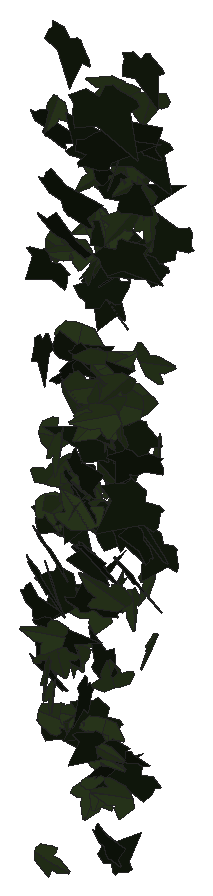
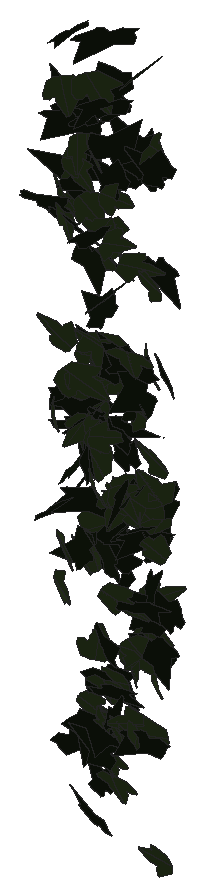
# SketchUp Ruby script. Lengths in inches.
U = 1.inch
M = Sketchup.active_model
def pt(a) = Geom::Point3d.new(a.map { |v| v * U })
def face(e, loops, mat)
  f = e.add_face(loops[0].map { |a| pt(a) })
  loops[1..].each { |l| e.add_face(l.map { |a| pt(a) }).erase! }
  f.material = f.back_material = mat if mat
  f
end
# faces: each face lists its corners as indices into pts; further lists are holes
def faces(e, pts, list, mat = nil) = list.each { |f| face(e, (f[0].is_a?(Array) ? f : [f]).map { |l| l.map { |i| pts[i] } }, mat) }
# xy, xz, yz: faces in a plane at the given z, y or x. An outline is a flat list of corners, or four numbers for a rectangle; further outlines are holes
def ring(l) = l.size == 4 ? [[l[0], l[1]], [l[2], l[1]], [l[2], l[3]], [l[0], l[3]]] : l.each_slice(2).to_a
def flat(e, list, mat, &to3) = list.each { |f| face(e, (f[0].is_a?(Array) ? f : [f]).map { |l| ring(l).map { |u, v| to3.(u, v) } }, mat) }
def xy(e, z, list, mat = nil) = flat(e, list, mat) { |x, y| [x, y, z] }
def xz(e, y, list, mat = nil) = flat(e, list, mat) { |x, z| [x, y, z] }
def yz(e, x, list, mat = nil) = flat(e, list, mat) { |y, z| [x, y, z] }
def lines(e, pts, list) = list.each { |a, b| e.add_line(pt(pts[a]), pt(pts[b])) }
# prism: a flat outline (further loops are holes) pulled along v
def prism(e, loops, v, mat = nil)
  f = face(e, loops, mat); d = Geom::Vector3d.new(v.map { |x| x * U })
  f.pushpull(f.normal.samedirection?(d) ? d.length : -d.length)
end
def box(e, o, s, mat = nil) = prism(e, [[o, [o[0] + s[0], o[1], o[2]], [o[0] + s[0], o[1] + s[1], o[2]], [o[0], o[1] + s[1], o[2]]]], [0, 0, s[2]], mat)
def at(x, y, z, deg = 0) = Geom::Transformation.translation(pt([x, y, z])) * Geom::Transformation.rotation(ORIGIN, Z_AXIS, deg.degrees)
def axes(o, x, y, z) = Geom::Transformation.new([*x, 0, *y, 0, *z, 0, *pt(o).to_a, 1])
def part(name) = M.definitions.add(name)
# library, detail: a bought-in or finely detailed component or shape, given as its bounding box
def library(name, o, s) = part(name).tap { |d| box(d.entities, o, s) }
def detail(e, o, s) = box(e.add_group.entities, o, s)
def put(e, d, t, mat = nil) = e.add_instance(d, t).tap { |i| i.material = mat if mat }
def group(e, t, mat = nil) = e.add_group.tap { |g| g.transformation = t; g.material = mat if mat }.entities
root = M.entities
M.materials.add("1026 AP 7946 SUNNY SIDE UP").color = [254, 231, 186]
M.materials.add("efeu1").color = [18, 25, 13]
M.materials.add("efeu2").color = [43, 57, 29]
c1 = part("ivyleaf_9")
p = [[1.54,2.16,1.25],[1.36,2.04,1.19],[-0.21,0.99,0.68],[-0.71,1.11,0.82],[-0.85,0.86,0.67],[-0.8,0.17,0.21],
  [-0.9,-0.01,0.1],[-0.67,-0.16,-0.02],[-0.08,-0.08,-0.05],[-0.03,-0.6,-0.4],[0.65,-0.88,-0.66],[0.83,-0.6,-0.49],
  [1.29,-0.42,-0.43],[1.8125,-0.07,-0.26],[1.21,0.44,0.15]]
faces(c1.entities,p,[[0,1,2,3,4,5,6,7,8,9,10,11,12,13,14]],"efeu1")
c2 = part("ivyleaf_10")
p = [[0,0.5,-0.03],[-0.0625,2.02,-0.43],[-0.19,2.01,-0.46],[-0.54,1.05,-0.29],[-0.52,0.625,-0.18],[-0.83,0.76,-0.28],
  [-1.16,0.64,-0.33],[-1.15,0.33,-0.24],[-0.77,-0.39,0.02],[-0.3,-0.51,0.16],[0.04,-0.48,0.23],[-0.02,2.01,-0.4375],
  [-0.06,2.01,-0.43],[0.04,-0.49,0.23],[0.67,-0.49,0.14],[1.38,0.36,-0.2],[1.375,0.51,-0.24],[0.81,0.65,-0.19],
  [0.62,0.59,-0.15],[0.6,1.09,-0.28],[0.5,1.23,-0.31]]
faces(c2.entities,p,[[0,1,2,3,4,5,6,7,8,9,10],[11,12,0,13,14,15,16,17,18,19,20]],"efeu2")
put(root,c1,axes([115.49,209.5,255.13],[-0.02705,-0.01002,-0.28667],[0.31242,-0.19569,-0.00654],[-0.30662,-0.19851,0.01862]),"1026 AP 7946 SUNNY SIDE UP")
put(root,c2,axes([114.77,209.6,259.99],[0.2251,-0.13197,0.25987],[0.25129,-0.19741,-0.2004],[0.37171,0.21338,-0.02189]),"1026 AP 7946 SUNNY SIDE UP")
put(root,c1,axes([114.3,209.47,257.21],[0.37652,-0.17867,-0.10207],[-0.14408,0.04077,-0.30679],[0.28627,0.25552,-0.02016]),"1026 AP 7946 SUNNY SIDE UP")
put(root,c1,axes([114.8,209.73,264.13],[0.4236,-0.17591,0.05148],[-0.04391,0.05014,0.33064],[-0.28462,-0.26955,0.02561]),"1026 AP 7946 SUNNY SIDE UP")
put(root,c1,axes([114.54,210.03,264.7],[-0.02289,-0.05893,0.36895],[0.34373,-0.28796,-0.0413],[0.45623,0.21399,0.04963]),"1026 AP 7946 SUNNY SIDE UP")
put(root,c1,axes([115.48,209.95,267.17],[-0.01242,-0.29597,-0.23302],[0.07302,0.22201,-0.3019],[0.57954,-0.03432,0.03305]),"1026 AP 7946 SUNNY SIDE UP")
put(root,c2,axes([114.04,210.18,254.74],[0.1255,-0.13859,0.23139],[0.21382,-0.18047,-0.16498],[0.3569,0.15685,0.01747]),"1026 AP 7946 SUNNY SIDE UP")
put(root,c2,axes([114.22,210.23,255.45],[-0.06096,-0.0694,-0.27227],[-0.3065,-0.17948,0.07708],[-0.30025,0.19731,-0.0234]),"1026 AP 7946 SUNNY SIDE UP")
put(root,c1,axes([115.21,209.97,265.93],[0.19681,0.10758,0.34086],[0.45934,0.1573,-0.16593],[-0.29545,0.31622,-0.03091]),"1026 AP 7946 SUNNY SIDE UP")
put(root,c2,axes([115.77,210.21,252.66],[0.15347,-0.06856,-0.24948],[-0.35736,0.08662,-0.11932],[0.16865,0.24593,-0.0258]),"1026 AP 7946 SUNNY SIDE UP")
put(root,c2,axes([115.29,210.39,260.32],[0.11174,0.03667,-0.27202],[-0.32658,-0.16404,-0.08195],[-0.2633,0.21903,-0.01379]),"1026 AP 7946 SUNNY SIDE UP")
put(root,c1,axes([116.04,210.45,258.76],[-0.41291,-0.14993,0.08346],[-0.08748,-0.06688,-0.31043],[0.25396,-0.26681,0.02877]),"1026 AP 7946 SUNNY SIDE UP")
put(root,c2,axes([115.51,210.35,256.59],[-0.27398,-0.02999,-0.24976],[-0.38052,-0.01791,0.18148],[-0.05045,0.29788,-0.01246]),"1026 AP 7946 SUNNY SIDE UP")
put(root,c1,axes([115.21,210.37,253.53],[0.09807,0.09154,-0.24899],[-0.17159,-0.21664,-0.11456],[-0.36922,0.12499,-0.01289]),"1026 AP 7946 SUNNY SIDE UP")
put(root,c2,axes([115.05,210.42,260.17],[0.26287,0.12848,-0.18106],[-0.19124,-0.12978,-0.21677],[-0.28504,0.20555,-0.02154]),"1026 AP 7946 SUNNY SIDE UP")
put(root,c2,axes([114.9,210.35,253.42],[-0.09458,-0.00259,-0.25397],[0.37678,-0.06028,-0.05993],[-0.09114,-0.24649,0.0158]),"1026 AP 7946 SUNNY SIDE UP")
put(root,c2,axes([114.94,210.43,263.36],[0.03486,-0.2653,-0.03718],[-0.00865,0.03424,-0.27405],[0.4206,0.02269,-0.00256]),"1026 AP 7946 SUNNY SIDE UP")
put(root,c1,axes([114.86,210.52,256.11],[0.33863,0.01352,0.15626],[-0.23931,0.02275,0.22076],[-0.00331,-0.26238,0.02564]),"1026 AP 7946 SUNNY SIDE UP")
put(root,c1,axes([115.53,210.38,263.84],[0.01179,-0.09483,-0.26226],[0.13606,0.24168,-0.0889],[0.40408,-0.07861,0.03759]),"1026 AP 7946 SUNNY SIDE UP")
put(root,c1,axes([115.07,210.59,251.21],[-0.02053,-0.0128,0.25407],[0.16189,-0.22485,-0.00772],[0.35309,0.10235,0.01831]),"1026 AP 7946 SUNNY SIDE UP")
put(root,c1,axes([113.72,210.6,254.33],[0.32164,-0.14094,-0.00848],[0.03041,0.01504,0.25487],[-0.21983,-0.20414,0.02286]),"1026 AP 7946 SUNNY SIDE UP")
put(root,c1,axes([113.82,210.49,255.3],[0.34152,0.05738,-0.19253],[0.26733,0.08346,0.23003],[0.15276,-0.27433,0.02789]),"1026 AP 7946 SUNNY SIDE UP")
put(root,c1,axes([113.64,210.67,256.93],[0.12988,-0.19391,0.19882],[0.1029,-0.18292,-0.21803],[0.41895,0.10504,-0.00808]),"1026 AP 7946 SUNNY SIDE UP")
put(root,c1,axes([115.83,210.7,257.8],[0.15212,-0.21561,-0.10881],[0.09876,-0.08582,0.24206],[-0.3635,-0.11354,0.02023]),"1026 AP 7946 SUNNY SIDE UP")
put(root,c1,axes([114.71,210.74,256.87],[0.1616,-0.23896,-0.11608],[0.08148,-0.09884,0.26727],[-0.40642,-0.11483,0.00743]),"1026 AP 7946 SUNNY SIDE UP")
put(root,c1,axes([113.84,210.53,262.95],[0.16397,0.01617,-0.24849],[-0.35536,-0.08702,-0.10713],[-0.13536,0.24804,-0.01975]),"1026 AP 7946 SUNNY SIDE UP")
put(root,c2,axes([113.72,210.74,254.05],[0.15207,-0.08677,0.24998],[0.24185,-0.18917,-0.13368],[0.32604,0.1808,-0.01744]),"1026 AP 7946 SUNNY SIDE UP")
put(root,c2,axes([114.01,210.55,254.86],[-0.26503,-0.20195,-0.05406],[0.07527,0.02672,-0.2701],[0.31887,-0.17415,0.01882]),"1026 AP 7946 SUNNY SIDE UP")
put(root,c1,axes([114.375,210.72,258.6],[-0.02097,0.02299,0.28356],[0.17416,-0.25185,0.02574],[0.39764,0.11152,0.00368]),"1026 AP 7946 SUNNY SIDE UP")
put(root,c2,axes([114.52,210.61,257.78],[0.28251,0.18577,0.10315],[-0.13701,-0.05295,0.26477],[0.30137,-0.19822,0.02368]),"1026 AP 7946 SUNNY SIDE UP")
put(root,c1,axes([113.3,210.73,255.48],[0.00996,0.00191,0.28312],[0.19716,-0.24462,-0.00265],[0.38452,0.12538,-0.00597]),"1026 AP 7946 SUNNY SIDE UP")
put(root,c1,axes([115.78,210.625,259.53],[0.14363,0.16281,-0.19678],[-0.11706,-0.17757,-0.19271],[-0.37804,0.11684,-0.01509]),"1026 AP 7946 SUNNY SIDE UP")
put(root,c1,axes([115.4,210.63,257.99],[0.19317,-0.16992,-0.17017],[-0.16403,0.12708,-0.21511],[0.3334,0.16097,-0.00723]),"1026 AP 7946 SUNNY SIDE UP")
put(root,c1,axes([113.93,210.66,255.84],[0.0528,-0.16787,0.18558],[-0.00367,0.18254,0.17583],[-0.38826,-0.02455,0.02358]),"1026 AP 7946 SUNNY SIDE UP")
put(root,c2,axes([114.875,210.75,253.59],[0.38898,0.00524,0.00305],[0.00537,-0.02319,-0.25391],[-0.00777,0.24631,-0.02251]),"1026 AP 7946 SUNNY SIDE UP")
put(root,c2,axes([114.84,210.8,260.14],[-0.24969,-0.2504,-0.08179],[-0.08858,-0.05646,0.30464],[-0.40276,0.16766,-0.0163]),"1026 AP 7946 SUNNY SIDE UP")
put(root,c1,axes([114.47,210.69,257.07],[0.39184,-0.07303,0.03452],[0.04122,-0.03074,-0.26675],[0.11973,0.24961,-0.02115]),"1026 AP 7946 SUNNY SIDE UP")
put(root,c1,axes([115.1,210.56,262.66],[-0.43965,0.1105,-0.05061],[-0.06013,0.03827,0.30917],[0.18082,0.28141,-0.02024]),"1026 AP 7946 SUNNY SIDE UP")
put(root,c2,axes([114.42,210.61,260.46],[-0.13007,-0.07676,0.26913],[0.25557,0.2057,0.1163],[-0.34432,0.18168,-0.01534]),"1026 AP 7946 SUNNY SIDE UP")
put(root,c2,axes([115.24,210.77,259.72],[-0.36298,0.15078,0.05464],[0.08607,-0.01136,0.28323],[0.23565,0.2364,-0.01929]),"1026 AP 7946 SUNNY SIDE UP")
put(root,c1,axes([113.37,210.9,260.95],[-0.14874,-0.02745,-0.25593],[0.37908,-0.0795,-0.08604],[-0.10277,-0.25351,0.05305]),"1026 AP 7946 SUNNY SIDE UP")
put(root,c2,axes([115.23,210.9,260.8],[-0.12716,-0.18939,0.17059],[-0.08336,-0.15835,-0.21281],[0.38783,-0.09613,0.01019]),"1026 AP 7946 SUNNY SIDE UP")
put(root,c2,axes([114.66,211,263.1],[0.01443,-0.03583,0.29115],[0.14207,-0.26801,-0.03957],[0.42515,0.09078,0.00334]),"1026 AP 7946 SUNNY SIDE UP")
put(root,c2,axes([113.38,210.89,250.3],[-0.0357,-0.01163,-0.24681],[0.32083,-0.12732,-0.0143],[-0.19808,-0.20413,0.02132]),"1026 AP 7946 SUNNY SIDE UP")
put(root,c1,axes([114.7,210.9,259.35],[-0.18541,-0.10774,-0.21597],[-0.24572,-0.13885,0.16372],[-0.27632,0.19576,-0.00067]),"1026 AP 7946 SUNNY SIDE UP")
put(root,c1,axes([115.65,210.9,267.59],[0.04255,-0.2644,-0.06219],[-0.01157,0.05842,-0.27346],[0.42576,0.02801,-0.00122]),"1026 AP 7946 SUNNY SIDE UP")
put(root,c1,axes([114.75,210.98,253.62],[-0.37392,-0.08956,0.05895],[-0.0713,-0.04271,-0.26091],[0.15162,-0.24095,0.02269]),"1026 AP 7946 SUNNY SIDE UP")
put(root,c2,axes([115.34,210.97,256.32],[0.2612,-0.09908,0.20455],[0.24482,-0.12567,-0.19896],[0.24974,0.22682,-0.0189]),"1026 AP 7946 SUNNY SIDE UP")
put(root,c1,axes([113.73,210.8125,254.89],[0.23732,0.07635,-0.22376],[-0.28899,-0.11732,-0.17439],[-0.21909,0.23744,-0.01234]),"1026 AP 7946 SUNNY SIDE UP")
put(root,c2,axes([114.68,211.01,259.58],[-0.02566,0.00037,0.29554],[0.36428,-0.16945,0.01281],[0.26604,0.23206,0.01097]),"1026 AP 7946 SUNNY SIDE UP")
put(root,c2,axes([114.05,210.97,254.79],[-0.22284,-0.18903,0.15562],[-0.10489,-0.13903,-0.24281],[0.36683,-0.15459,0.0251]),"1026 AP 7946 SUNNY SIDE UP")
put(root,c1,axes([113.85,211.07,267.32],[-0.01384,-0.29289,0.11753],[-0.00898,-0.11563,-0.30254],[0.49512,-0.01029,-0.0022]),"1026 AP 7946 SUNNY SIDE UP")
put(root,c2,axes([114.27,210.8,257.76],[0.03886,-0.25967,0.13505],[-0.02362,0.13174,0.26948],[-0.45784,-0.02884,-0.00244]),"1026 AP 7946 SUNNY SIDE UP")
put(root,c1,axes([113.9375,211.03,260.02],[0.11703,-0.16173,0.19744],[0.10624,-0.18058,-0.1842],[0.38088,0.10006,-0.00928]),"1026 AP 7946 SUNNY SIDE UP")
put(root,c1,axes([115.42,210.98,265.85],[-0.14077,0.00313,0.31162],[0.29124,-0.24882,0.05768],[0.37604,0.19388,0.07199]),"1026 AP 7946 SUNNY SIDE UP")
put(root,c1,axes([115.99,210.93,263.52],[-0.41705,0.07773,0.04163],[-0.07052,-0.01141,-0.28378],[-0.11797,-0.26798,0.02245]),"1026 AP 7946 SUNNY SIDE UP")
put(root,c1,axes([115.45,210.78,258.78],[0.06346,-0.01232,-0.27237],[-0.40423,0.06151,-0.04303],[0.09855,0.26021,-0.00112]),"1026 AP 7946 SUNNY SIDE UP")
put(root,c1,axes([114.58,210.98,259.4],[-0.15853,-0.07114,-0.29029],[0.43716,0.06184,-0.11837],[0.13101,-0.29243,0.0437]),"1026 AP 7946 SUNNY SIDE UP")
put(root,c2,axes([115.83,211.01,255.57],[0.16067,-0.22447,0.10209],[0.04915,-0.09595,-0.25441],[0.3835,0.10634,-0.01016]),"1026 AP 7946 SUNNY SIDE UP")
put(root,c1,axes([114.4,211.03,257.99],[-0.38232,-0.06635,0.01689],[-0.01411,-0.03044,-0.25833],[0.10668,-0.24181,0.02634]),"1026 AP 7946 SUNNY SIDE UP")
put(root,c2,axes([114.99,211.06,265.32],[0.23828,-0.2311,0.14184],[0.09771,-0.12522,-0.28502],[0.41263,0.1631,-0.01441]),"1026 AP 7946 SUNNY SIDE UP")
put(root,c1,axes([114.04,211.12,258.13],[0.07279,-0.22922,0.19791],[0.10446,-0.183,-0.24089],[0.45988,0.07785,0.02339]),"1026 AP 7946 SUNNY SIDE UP")
put(root,c2,axes([115.16,211.06,264.08],[-0.10995,-0.23584,0.15375],[-0.04715,-0.148,-0.25401],[0.43744,-0.07523,0.01127]),"1026 AP 7946 SUNNY SIDE UP")
put(root,c2,axes([114.97,210.99,256.28],[0.06811,-0.24122,-0.05295],[0.01955,-0.04859,0.25217],[-0.38688,-0.04492,0.00342]),"1026 AP 7946 SUNNY SIDE UP")
put(root,c2,axes([114.93,211.02,254.38],[-0.22262,-0.21073,-0.08641],[-0.09051,-0.0608,0.26083],[-0.34424,0.15226,-0.0127]),"1026 AP 7946 SUNNY SIDE UP")
put(root,c1,axes([114.57,211.02,265.31],[0.17266,0.08014,0.27824],[-0.42051,-0.05999,0.13022],[0.13712,-0.28489,0.04898]),"1026 AP 7946 SUNNY SIDE UP")
put(root,c2,axes([114.69,210.98,252.2],[0.38337,-0.03766,-0.00505],[-0.01271,-0.02175,-0.2532],[0.05831,0.24289,-0.02199]),"1026 AP 7946 SUNNY SIDE UP")
put(root,c2,axes([114.82,210.94,261.13],[-0.43336,-0.1602,0.00947],[0.00821,-0.02901,-0.32734],[0.25227,-0.27426,0.02693]),"1026 AP 7946 SUNNY SIDE UP")
put(root,c2,axes([114.14,211.04,263.08],[0.08868,0.04076,-0.25751],[-0.34943,-0.11537,-0.07165],[-0.19178,0.22906,0.01146]),"1026 AP 7946 SUNNY SIDE UP")
put(root,c2,axes([113.74,211.13,257.68],[0.0458,0.00598,0.30893],[0.33534,-0.21222,-0.01822],[0.33155,0.21382,-0.02424]),"1026 AP 7946 SUNNY SIDE UP")
put(root,c2,axes([115.4375,211.14,264.97],[-0.01451,-0.0973,0.25221],[-0.03917,-0.2441,-0.10211],[0.41319,-0.02656,-0.00082]),"1026 AP 7946 SUNNY SIDE UP")
put(root,c2,axes([113.55,211.08,265.88],[0.05555,0.17276,-0.19862],[-0.05516,-0.19059,-0.18276],[-0.40446,0.04972,-0.00235]),"1026 AP 7946 SUNNY SIDE UP")
put(root,c2,axes([113.54,210.92,258.17],[-0.22673,-0.22982,0.10839],[0.06704,0.0988,0.27964],[-0.39262,0.14959,-0.01484]),"1026 AP 7946 SUNNY SIDE UP")
put(root,c1,axes([115.22,211.07,259.76],[-0.20547,-0.27009,-0.10705],[0.11587,0.07747,-0.30701],[0.43914,-0.14681,0.03092]),"1026 AP 7946 SUNNY SIDE UP")
put(root,c1,axes([114.37,211.03,260.6875],[-0.01217,-0.03991,0.32018],[0.37269,-0.20444,-0.02214],[0.32281,0.23452,0.03763]),"1026 AP 7946 SUNNY SIDE UP")
put(root,c2,axes([114.78,211.06,258.43],[-0.24243,0.02516,0.27815],[0.39951,-0.09465,0.15808],[0.14834,0.29603,0.02883]),"1026 AP 7946 SUNNY SIDE UP")
put(root,c2,axes([113.35,211.06,258.98],[0.11121,-0.09124,-0.25557],[0.31765,-0.14614,0.11408],[-0.26685,-0.21198,0.02929]),"1026 AP 7946 SUNNY SIDE UP")
put(root,c2,axes([113.74,210.9,257.65],[-0.15981,-0.22365,0.154],[0.08022,0.14226,0.25367],[-0.41644,0.11323,-0.01023]),"1026 AP 7946 SUNNY SIDE UP")
put(root,c2,axes([115.75,210.98,263.79],[0.04522,-0.32358,-0.03934],[-0.00781,0.03605,-0.33445],[0.51194,0.02913,-0.00163]),"1026 AP 7946 SUNNY SIDE UP")
put(root,c2,axes([114.41,210.93,257.86],[-0.27789,-0.2432,-0.10064],[0.11522,0.06554,-0.30866],[0.39484,-0.1903,0.01924]),"1026 AP 7946 SUNNY SIDE UP")
put(root,c2,axes([113.47,210.9375,257.66],[0.15255,0.23441,0.05157],[0.04697,0.04031,-0.26082],[-0.37352,0.1008,-0.01174]),"1026 AP 7946 SUNNY SIDE UP")
put(root,c1,axes([115.46,210.99,265.8],[-0.10589,-0.18942,-0.25154],[0.21007,0.20629,-0.20252],[0.43668,-0.14517,0.03643]),"1026 AP 7946 SUNNY SIDE UP")
put(root,c1,axes([113.3125,211.07,265.33],[0.11124,-0.0536,0.25227],[0.2767,-0.17103,-0.09183],[0.28136,0.18939,-0.00943]),"1026 AP 7946 SUNNY SIDE UP")
put(root,c1,axes([114.61,210.9,256.37],[-0.05128,0.26947,0.06962],[-0.00927,-0.06716,0.27889],[0.43616,0.03025,0.01411]),"1026 AP 7946 SUNNY SIDE UP")
put(root,c2,axes([113.8,211.15,260.04],[-0.05751,0.01978,-0.31945],[0.31116,-0.23938,-0.04116],[-0.3769,-0.20065,0.01476]),"1026 AP 7946 SUNNY SIDE UP")
put(root,c2,axes([114.46,210.98,252.84],[0.09081,0.02675,0.24506],[0.36763,0.04547,-0.06352],[-0.07965,0.24038,-0.01378]),"1026 AP 7946 SUNNY SIDE UP")
put(root,c2,axes([115.02,211.07,266.77],[-0.33911,-0.16557,0.14113],[-0.15081,-0.101,-0.27998],[0.30344,-0.23523,0.01857]),"1026 AP 7946 SUNNY SIDE UP")
put(root,c2,axes([115.25,211.17,260.14],[-0.07737,-0.06551,-0.30276],[-0.36791,-0.17851,0.08041],[-0.29708,0.23813,-0.02073]),"1026 AP 7946 SUNNY SIDE UP")
put(root,c2,axes([114.81,210.93,260.95],[0.28785,0.00144,-0.19508],[0.29055,0.05634,0.18478],[0.06523,-0.25729,0.03779]),"1026 AP 7946 SUNNY SIDE UP")
put(root,c1,axes([113.97,211.03,260.73],[-0.10792,0.01566,0.29636],[0.37296,-0.16464,0.06659],[0.2569,0.24559,0.02783]),"1026 AP 7946 SUNNY SIDE UP")
put(root,c2,axes([114.13,210.92,258.27],[-0.1984,-0.17657,-0.20026],[0.22258,0.13462,-0.22097],[0.34643,-0.18761,0.02728]),"1026 AP 7946 SUNNY SIDE UP")
put(root,c1,axes([115.2,210.92,264.55],[0.01545,0.01948,0.33278],[0.50774,0.01911,-0.01119],[-0.03101,0.3225,-0.01754]),"1026 AP 7946 SUNNY SIDE UP")
put(root,c1,axes([114.91,211,250.68],[-0.16141,0.18303,0.17152],[0.15144,-0.13526,0.21492],[0.35718,0.14006,-0.01361]),"1026 AP 7946 SUNNY SIDE UP")
put(root,c1,axes([114.57,211.29,262.24],[-0.07987,-0.2511,0.18277],[-0.02279,-0.17911,-0.26436],[0.48421,-0.04985,0.01771]),"1026 AP 7946 SUNNY SIDE UP")
put(root,c1,axes([114.64,211.03,266.41],[0.01762,-0.23886,-0.21277],[0.06406,0.20468,-0.24198],[0.49096,-0.01813,0.03921]),"1026 AP 7946 SUNNY SIDE UP")
put(root,c1,axes([114.41,211.21,253.0625],[0.01892,0.04229,0.25577],[-0.18178,-0.21963,0.04307],[0.35141,-0.11589,0.00851]),"1026 AP 7946 SUNNY SIDE UP")
put(root,c1,axes([115.1,210.92,262.95],[-0.00003,0.26393,0.01852],[0.00005,0.01648,-0.27181],[-0.41582,-0.00001,-0.00003]),"1026 AP 7946 SUNNY SIDE UP")
put(root,c2,axes([114.8,211,263.56],[0.38169,0.05373,0.08797],[-0.14437,0.02728,0.25224],[0.06477,-0.25577,0.04381]),"1026 AP 7946 SUNNY SIDE UP")
put(root,c1,axes([114.29,211.18,264.79],[0.09394,-0.05292,0.27331],[0.22753,-0.22367,-0.08075],[0.35997,0.15519,-0.02029]),"1026 AP 7946 SUNNY SIDE UP")
put(root,c2,axes([114.53,211.04,255.76],[0.17015,-0.04936,-0.28896],[-0.42666,0.07229,-0.12064],[0.13459,0.29155,-0.01714]),"1026 AP 7946 SUNNY SIDE UP")
put(root,c2,axes([113.375,211.1875,262.9],[-0.02226,-0.0389,-0.26243],[0.27728,-0.18719,0.01827],[-0.29499,-0.17302,0.03698]),"1026 AP 7946 SUNNY SIDE UP")
put(root,c2,axes([115.5,211.08,264.84],[-0.3004,-0.01174,0.18764],[-0.28172,-0.03874,-0.19633],[0.05529,-0.26114,0.01912]),"1026 AP 7946 SUNNY SIDE UP")
put(root,c1,axes([115.35,211.22,252.51],[0.01161,-0.00532,-0.26424],[-0.15122,-0.23792,0.00084],[-0.37394,0.09605,-0.00855]),"1026 AP 7946 SUNNY SIDE UP")
put(root,c1,axes([114.97,211.03,257.74],[0.03081,-0.1384,-0.28678],[0.19737,0.25789,-0.12182],[0.44601,-0.10456,0.07372]),"1026 AP 7946 SUNNY SIDE UP")
put(root,c2,axes([114.35,211.15,251.85],[0.40012,-0.04245,-0.00458],[-0.01258,-0.02252,-0.2648],[0.06589,0.2535,-0.02276]),"1026 AP 7946 SUNNY SIDE UP")
put(root,c2,axes([115.53,211.23,264.19],[0.29502,-0.11111,0.20435],[0.24873,-0.12208,-0.22459],[0.258,0.24474,-0.01716]),"1026 AP 7946 SUNNY SIDE UP")
put(root,c2,axes([113.76,211.29,253.03],[-0.03329,-0.11713,-0.22662],[-0.01173,-0.21971,0.12034],[-0.39077,0.01657,0.0157]),"1026 AP 7946 SUNNY SIDE UP")
put(root,c2,axes([115.3,211.09,265.36],[-0.06309,-0.27148,-0.06678],[0.04158,0.05994,-0.28182],[0.43634,-0.04496,0.0172]),"1026 AP 7946 SUNNY SIDE UP")
put(root,c2,axes([114.07,211.15,258.2],[-0.35428,-0.13699,0.09073],[-0.09661,-0.06915,-0.27076],[0.23787,-0.23211,0.02516]),"1026 AP 7946 SUNNY SIDE UP")
put(root,c1,axes([113.79,211.26,255.9],[-0.35089,-0.15795,-0.0066],[0.02663,-0.01442,-0.28086],[0.24708,-0.22276,0.0209]),"1026 AP 7946 SUNNY SIDE UP")
put(root,c2,axes([115.32,211.25,260.36],[-0.24659,-0.12262,0.26317],[-0.25921,-0.19896,-0.20325],[0.36361,-0.22499,0.03358]),"1026 AP 7946 SUNNY SIDE UP")
put(root,c1,axes([115.18,211.35,259.37],[-0.13643,-0.17053,0.18817],[-0.08478,-0.17706,-0.19669],[0.38481,-0.09947,0.02338]),"1026 AP 7946 SUNNY SIDE UP")
put(root,c2,axes([114.69,211.3,259.26],[-0.00856,0.0021,0.26187],[-0.17278,-0.22927,-0.00181],[0.36041,-0.10986,0.00535]),"1026 AP 7946 SUNNY SIDE UP")
put(root,c1,axes([114.58,211.03,252.34],[0.15191,0.2434,-0.0416],[-0.00568,0.04624,0.26925],[0.38828,-0.09455,0.02022]),"1026 AP 7946 SUNNY SIDE UP")
put(root,c2,axes([114.42,211.13,252.87],[0.3598,-0.09872,-0.07263],[0.1154,-0.0057,0.25561],[-0.15124,-0.2392,0.02225]),"1026 AP 7946 SUNNY SIDE UP")
put(root,c1,axes([114.8,211.23,263.64],[-0.04299,-0.27397,-0.08805],[0.02294,0.08285,-0.28309],[0.44996,-0.0304,0.00602]),"1026 AP 7946 SUNNY SIDE UP")
put(root,c2,axes([113.36,211.08,253.12],[0.05824,0.02873,0.26307],[0.35073,0.12418,-0.04703],[-0.20012,0.226,-0.00586]),"1026 AP 7946 SUNNY SIDE UP")
put(root,c2,axes([113.77,211.26,254.34],[-0.1076,0.0755,0.22218],[0.2743,-0.12745,0.10245],[0.23107,0.18646,-0.01815]),"1026 AP 7946 SUNNY SIDE UP")
put(root,c1,axes([113.54,211.15,257.45],[-0.0046,-0.22727,-0.2097],[0.08673,0.19853,-0.22946],[0.47046,-0.03882,0.04025]),"1026 AP 7946 SUNNY SIDE UP")
put(root,c2,axes([114.37,211.34,264.62],[-0.04964,-0.12907,0.22934],[-0.0518,-0.22116,-0.13775],[0.4023,-0.0444,0.01056]),"1026 AP 7946 SUNNY SIDE UP")
put(root,c1,axes([114.97,211.22,256.6875],[0.32515,-0.17115,0.08127],[0.07433,-0.06774,-0.27606],[0.28751,0.21106,-0.02053]),"1026 AP 7946 SUNNY SIDE UP")
put(root,c1,axes([115.74,211.39,257.36],[-0.15154,-0.23742,0.13564],[-0.06327,-0.12712,-0.26454],[0.42322,-0.10402,0.00902]),"1026 AP 7946 SUNNY SIDE UP")
put(root,c1,axes([114.8125,211.07,252.84],[0.34882,0.15794,-0.07219],[-0.07019,-0.05928,-0.27999],[-0.26306,0.22524,-0.02102]),"1026 AP 7946 SUNNY SIDE UP")
put(root,c1,axes([114.73,211.03,254.5625],[0.02436,0.00626,0.27347],[-0.1381,0.25103,0.00065],[-0.39396,-0.08761,0.01669]),"1026 AP 7946 SUNNY SIDE UP")
put(root,c2,axes([113.26,211.18,257.18],[-0.17082,0.01597,0.25362],[0.38516,0.03824,0.10906],[-0.04506,0.26628,-0.02928]),"1026 AP 7946 SUNNY SIDE UP")
put(root,c2,axes([114.51,211.21,253.2],[0.32821,-0.13495,-0.04915],[-0.0806,0.00684,-0.25504],[0.20971,0.21383,-0.02111]),"1026 AP 7946 SUNNY SIDE UP")
put(root,c2,axes([113.96,211.22,261.25],[0.40663,0.03266,-0.0066],[-0.0053,-0.02569,-0.26744],[-0.05212,0.25741,-0.02431]),"1026 AP 7946 SUNNY SIDE UP")
put(root,c1,axes([115.13,210.97,258.42],[-0.01489,0.00291,0.31762],[0.11418,0.29978,0.00114],[-0.47115,0.07256,-0.00976]),"1026 AP 7946 SUNNY SIDE UP")
put(root,c2,axes([113.71,211.22,254.72],[0.30667,0.03192,0.14444],[0.22339,-0.00828,-0.20196],[-0.03308,0.23995,-0.02476]),"1026 AP 7946 SUNNY SIDE UP")
put(root,c2,axes([115.57,211.25,256.65],[0.24611,-0.229,0.00407],[-0.01203,-0.01158,-0.28551],[0.35997,0.15618,-0.01232]),"1026 AP 7946 SUNNY SIDE UP")
put(root,c1,axes([114.44,211.38,262.03],[0.10244,-0.17396,0.22316],[0.13795,-0.1993,-0.19236],[0.41578,0.10899,0.00884]),"1026 AP 7946 SUNNY SIDE UP")
put(root,c1,axes([116.2,211.16,263.8],[-0.42804,-0.07852,-0.05081],[-0.08557,0.01315,0.29059],[-0.11759,0.27626,-0.02652]),"1026 AP 7946 SUNNY SIDE UP")
put(root,c1,axes([113.85,211.39,257.5],[-0.17713,-0.22344,0.05887],[-0.02186,-0.05832,-0.25775],[0.36249,-0.1127,0.01323]),"1026 AP 7946 SUNNY SIDE UP")
put(root,c1,axes([113.55,211.18,253.04],[-0.06328,-0.09585,-0.23586],[0.18841,0.19498,-0.10491],[0.34087,-0.12557,0.0142]),"1026 AP 7946 SUNNY SIDE UP")
put(root,c2,axes([114.32,211.4,263.66],[0.07284,0.10032,-0.2527],[-0.21202,-0.20611,-0.11402],[-0.35969,0.14181,0.01604]),"1026 AP 7946 SUNNY SIDE UP")
put(root,c2,axes([115.65,211.39,259.42],[0.10902,-0.0848,0.22402],[0.22584,-0.16395,-0.11375],[0.29019,0.15945,0.00436]),"1026 AP 7946 SUNNY SIDE UP")
put(root,c1,axes([114.09,211.12,258.3],[0.12635,-0.13415,-0.26446],[-0.25077,0.20095,-0.15891],[0.37892,0.17772,-0.01699]),"1026 AP 7946 SUNNY SIDE UP")
put(root,c2,axes([115.1,211.15,259.37],[-0.17912,-0.18315,-0.17553],[0.17308,0.13016,-0.22054],[0.35198,-0.15721,0.01912]),"1026 AP 7946 SUNNY SIDE UP")
put(root,c2,axes([113.82,211.125,253.26],[0.02503,0.02111,0.24339],[0.24291,0.1786,-0.02614],[-0.28277,0.15529,-0.0009]),"1026 AP 7946 SUNNY SIDE UP")
put(root,c2,axes([115.45,211.28,261.08],[-0.20665,0.01984,0.25206],[0.38533,-0.00313,0.13591],[0.01911,0.27761,-0.01485]),"1026 AP 7946 SUNNY SIDE UP")
put(root,c2,axes([115.54,211.28,266.62],[-0.27166,-0.23787,0.03648],[-0.01249,-0.03959,-0.30261],[0.37826,-0.17214,0.01621]),"1026 AP 7946 SUNNY SIDE UP")
put(root,c2,axes([114.82,211.43,259.42],[-0.00127,0.03419,-0.25306],[-0.03701,-0.24474,-0.03641],[-0.38852,0.0232,0.00429]),"1026 AP 7946 SUNNY SIDE UP")
put(root,c1,axes([113.77,211.01,260.44],[0.17273,0.18064,0.22242],[0.18282,0.18075,-0.21671],[-0.40177,0.15991,-0.00299]),"1026 AP 7946 SUNNY SIDE UP")
put(root,c2,axes([114.65,211.39,258.22],[0.26013,-0.13927,0.17498],[0.17503,-0.13129,-0.22233],[0.29886,0.19812,-0.02209]),"1026 AP 7946 SUNNY SIDE UP")
